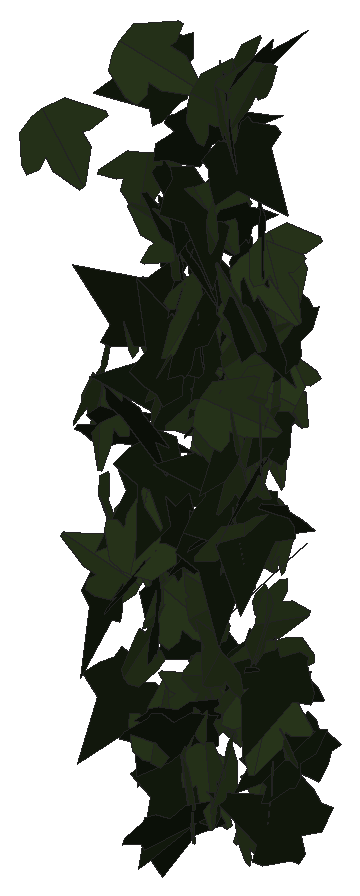
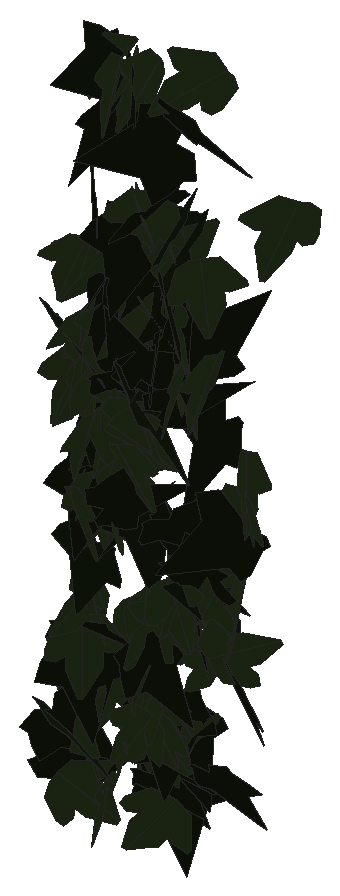
# SketchUp Ruby script. Lengths in inches.
U = 1.inch
M = Sketchup.active_model
def pt(a) = Geom::Point3d.new(a.map { |v| v * U })
def face(e, loops, mat)
  f = e.add_face(loops[0].map { |a| pt(a) })
  loops[1..].each { |l| e.add_face(l.map { |a| pt(a) }).erase! }
  f.material = f.back_material = mat if mat
  f
end
# faces: each face lists its corners as indices into pts; further lists are holes
def faces(e, pts, list, mat = nil) = list.each { |f| face(e, (f[0].is_a?(Array) ? f : [f]).map { |l| l.map { |i| pts[i] } }, mat) }
# xy, xz, yz: faces in a plane at the given z, y or x. An outline is a flat list of corners, or four numbers for a rectangle; further outlines are holes
def ring(l) = l.size == 4 ? [[l[0], l[1]], [l[2], l[1]], [l[2], l[3]], [l[0], l[3]]] : l.each_slice(2).to_a
def flat(e, list, mat, &to3) = list.each { |f| face(e, (f[0].is_a?(Array) ? f : [f]).map { |l| ring(l).map { |u, v| to3.(u, v) } }, mat) }
def xy(e, z, list, mat = nil) = flat(e, list, mat) { |x, y| [x, y, z] }
def xz(e, y, list, mat = nil) = flat(e, list, mat) { |x, z| [x, y, z] }
def yz(e, x, list, mat = nil) = flat(e, list, mat) { |y, z| [x, y, z] }
def lines(e, pts, list) = list.each { |a, b| e.add_line(pt(pts[a]), pt(pts[b])) }
# prism: a flat outline (further loops are holes) pulled along v
def prism(e, loops, v, mat = nil)
  f = face(e, loops, mat); d = Geom::Vector3d.new(v.map { |x| x * U })
  f.pushpull(f.normal.samedirection?(d) ? d.length : -d.length)
end
def box(e, o, s, mat = nil) = prism(e, [[o, [o[0] + s[0], o[1], o[2]], [o[0] + s[0], o[1] + s[1], o[2]], [o[0], o[1] + s[1], o[2]]]], [0, 0, s[2]], mat)
def at(x, y, z, deg = 0) = Geom::Transformation.translation(pt([x, y, z])) * Geom::Transformation.rotation(ORIGIN, Z_AXIS, deg.degrees)
def axes(o, x, y, z) = Geom::Transformation.new([*x, 0, *y, 0, *z, 0, *pt(o).to_a, 1])
def part(name) = M.definitions.add(name)
# library, detail: a bought-in or finely detailed component or shape, given as its bounding box
def library(name, o, s) = part(name).tap { |d| box(d.entities, o, s) }
def detail(e, o, s) = box(e.add_group.entities, o, s)
def put(e, d, t, mat = nil) = e.add_instance(d, t).tap { |i| i.material = mat if mat }
def group(e, t, mat = nil) = e.add_group.tap { |g| g.transformation = t; g.material = mat if mat }.entities
root = M.entities
M.materials.add("efeu1").color = [18, 25, 13]
M.materials.add("efeu2").color = [43, 57, 29]
c1 = part("ivyleaf_9")
p = [[1.54,2.16,1.25],[1.36,2.04,1.19],[-0.21,0.99,0.68],[-0.71,1.11,0.82],[-0.85,0.86,0.67],[-0.8,0.17,0.21],
  [-0.9,-0.01,0.1],[-0.67,-0.16,-0.02],[-0.08,-0.08,-0.05],[-0.03,-0.6,-0.4],[0.65,-0.88,-0.66],[0.83,-0.6,-0.49],
  [1.29,-0.42,-0.43],[1.8125,-0.07,-0.26],[1.21,0.44,0.15]]
faces(c1.entities,p,[[0,1,2,3,4,5,6,7,8,9,10,11,12,13,14]],"efeu1")
c2 = part("ivyleaf_10")
p = [[0,0.5,-0.03],[-0.0625,2.02,-0.43],[-0.19,2.01,-0.46],[-0.54,1.05,-0.29],[-0.52,0.625,-0.18],[-0.83,0.76,-0.28],
  [-1.16,0.64,-0.33],[-1.15,0.33,-0.24],[-0.77,-0.39,0.02],[-0.3,-0.51,0.16],[0.04,-0.48,0.23],[-0.02,2.01,-0.4375],
  [-0.06,2.01,-0.43],[0.04,-0.49,0.23],[0.67,-0.49,0.14],[1.38,0.36,-0.2],[1.375,0.51,-0.24],[0.81,0.65,-0.19],
  [0.62,0.59,-0.15],[0.6,1.09,-0.28],[0.5,1.23,-0.31]]
faces(c2.entities,p,[[0,1,2,3,4,5,6,7,8,9,10],[11,12,0,13,14,15,16,17,18,19,20]],"efeu2")
put(root,c1,axes([597.17,133.51,184.68],[0.19344,0.78927,-0.31319],[-0.07682,-0.30363,-0.81262],[-0.84566,0.20812,0.00218]))
put(root,c1,axes([597.22,133.8,197.03],[-0.33074,-0.73089,0.28254],[0.11402,0.25853,0.80224],[-0.77526,0.34984,-0.00255]))
put(root,c2,axes([598.65,133.66,205.125],[-0.33147,0.76317,-0.05677],[0.02262,-0.05207,-0.83204],[-0.76494,-0.33224,-0.00001]))
put(root,c1,axes([598.06,134.29,192.28],[0.09224,-0.89011,0.23083],[0.02783,-0.22918,-0.89487],[0.91914,0.09626,0.00393]))
put(root,c2,axes([596.73,133.97,196.96],[0.36238,-0.84765,0.07309],[0.03386,-0.06501,-0.92184],[0.85012,0.36391,0.00557]))
put(root,c1,axes([595.71,133.54,195.63],[0.79787,0.04653,-0.34518],[-0.34406,-0.02892,-0.79918],[-0.05418,0.86885,-0.00812]))
put(root,c2,axes([596.19,133.4,205.63],[0.32603,0.37985,0.79426],[0.47436,0.63773,-0.49971],[-0.7417,0.57484,0.02954]))
put(root,c1,axes([598.14,134.25,204.97],[0.01634,-0.07031,-0.84134],[0.83164,-0.14369,0.02816],[-0.14551,-0.82914,0.06646]))
put(root,c1,axes([598.95,134.2,193.69],[-0.38224,-0.75949,-0.28995],[0.16171,0.24297,-0.8496],[0.79671,-0.41369,0.03334]))
put(root,c2,axes([599.41,133.78,198.8],[-0.68374,0.33028,-0.53436],[-0.48633,0.22162,0.75927],[0.39762,0.839,0.0098]))
put(root,c2,axes([597.57,134.4,201.07],[0.01121,-0.17778,-0.85341],[0.47011,-0.7175,0.15564],[-0.7341,-0.4622,0.08664]))
put(root,c2,axes([593.4375,133.54,202.57],[0.43362,0.73756,0.41788],[0.06795,0.43763,-0.84292],[-0.84499,0.41369,0.14666]))
put(root,c1,axes([596.05,134.34,197.8],[0.16484,0.03859,0.90855],[-0.8719,-0.2556,0.16904],[0.25833,-0.8873,-0.00918]))
put(root,c2,axes([596.96,134.32,200.34],[-0.49306,-0.19256,-0.65801],[-0.57053,-0.33422,0.52531],[-0.3802,0.75125,0.06504]))
put(root,c2,axes([595.79,133.85,191.36],[0.8262,0.16039,-0.09412],[0.09089,0.02566,0.84159],[0.16224,-0.83115,0.00782]))
put(root,c2,axes([598.23,133.4,205.06],[0.01695,0.52,0.68475],[-0.19293,0.66972,-0.50381],[-0.83789,-0.14369,0.12985]))
put(root,c2,axes([599.07,133.98,193.07],[-0.43575,-0.80714,-0.07981],[0.04881,0.06434,-0.91717],[0.8096,-0.43831,0.01234]))
put(root,c2,axes([599.13,134.33,205.61],[-0.08859,-0.71936,0.36185],[-0.03531,-0.36021,-0.72475],[0.80446,-0.09503,0.00804]))
put(root,c2,axes([596.08,133.56,188.625],[0.1876,-0.54419,0.68042],[-0.2028,0.64962,0.57548],[-0.84734,-0.27596,0.01291]))
put(root,c1,axes([599.04,133.74,203.9],[0.12591,-0.45757,-0.69364],[-0.21384,0.66008,-0.47425],[0.80298,0.24754,-0.01753]))
put(root,c1,axes([596.8,134.53,196.1],[-0.32515,-0.07178,0.756],[-0.67039,-0.3592,-0.32243],[0.35674,-0.74043,0.08313]))
put(root,c2,axes([598.5625,133.56,196.59],[0.31512,0.26551,0.76924],[0.35454,0.69771,-0.38606],[-0.73249,0.45193,0.14408]))
put(root,c1,axes([596.55,134.64,201.24],[0.09239,-0.56269,0.59128],[0.12989,-0.57733,-0.56972],[0.80583,0.15758,0.02404]))
put(root,c1,axes([599.37,134.23,194.88],[-0.46831,0.47847,-0.45991],[0.30892,-0.34103,-0.66935],[-0.58738,-0.56083,0.01465]))
put(root,c1,axes([597.77,133.64,197.98],[-0.25926,0.53962,0.66936],[-0.4009,0.5426,-0.59271],[-0.76059,-0.46993,0.08425]))
put(root,c1,axes([596.28,134.29,200.88],[0.65973,-0.63387,0.08771],[0.06311,-0.06091,-0.9149],[0.63679,0.66274,-0.00019]))
put(root,c2,axes([598.71,134.17,195.99],[-0.30812,0.74007,-0.17715],[0.07386,-0.16113,-0.80163],[-0.75738,-0.31679,-0.00611]))
put(root,c1,axes([596.51,133.78,190.06],[-0.16401,0.14057,-0.81785],[-0.80945,0.15657,0.18924],[0.18283,0.81931,0.10416]))
put(root,c2,axes([597.125,134.18,185.7],[-0.52445,0.67905,-0.13617],[-0.00111,-0.17162,-0.85161],[-0.69257,-0.51394,0.10447]))
put(root,c2,axes([597.5,134.34,186.07],[0.67909,-0.21797,0.37866],[0.38147,-0.0454,-0.71026],[0.21301,0.77619,0.06479]))
put(root,c1,axes([596.69,134.18,186.85],[0.11997,0.66516,-0.5349],[-0.16394,-0.51214,-0.67363],[-0.83766,0.19549,0.05523]))
put(root,c2,axes([598.03,134.75,186.15],[-0.08182,0.24007,-0.78209],[0.1356,-0.77114,-0.2509],[-0.80679,-0.15396,0.03714]))
put(root,c2,axes([598.3125,134.55,192.98],[0.31203,-0.41931,0.67242],[0.65243,-0.27426,-0.47377],[0.44979,0.68869,0.22074]))
put(root,c2,axes([598.28,134.04,189.34],[-0.6344,0.11559,0.54828],[-0.53924,0.09913,-0.64485],[-0.15228,-0.83262,-0.00066]))
put(root,c1,axes([596.93,134.62,185.24],[-0.76967,-0.37313,-0.11884],[0.1206,0.02348,-0.85478],[0.37257,-0.77843,0.03118]))
put(root,c2,axes([599.02,133.86,194.97],[-0.0018,-0.64385,-0.59161],[0.02941,0.59123,-0.64353],[0.87389,-0.02122,0.02044]))
put(root,c1,axes([595.53,133.67,190.4],[-0.24967,0.76452,-0.27388],[-0.08823,0.2593,0.80425],[0.80729,0.26478,0.00319]))
put(root,c1,axes([597.36,134.59,201.79],[0.02343,-0.83752,-0.09939],[-0.00566,0.09927,-0.83785],[0.84338,0.02394,-0.00286]))
put(root,c1,axes([598.03,133.96,192.67],[-0.15279,0.91899,-0.03563],[0.00123,-0.03592,-0.93159],[-0.91968,-0.15273,0.00467]))
put(root,c2,axes([597.34,134.62,198.8],[0.35778,0.60825,-0.53666],[-0.33189,-0.42542,-0.70344],[-0.74014,0.48479,0.05602]))
put(root,c1,axes([596.59,134.4,204.74],[-0.73716,0.29395,0.34517],[-0.33352,0.0947,-0.79294],[-0.3071,-0.80844,0.03261]))
put(root,c2,axes([597.92,134.39,195.93],[-0.53778,-0.74544,-0.00437],[0.00148,0.00432,-0.91918],[0.74545,-0.53778,-0.00132]))
put(root,c1,axes([598.88,134.2,199.23],[0.53349,-0.5158,-0.46393],[-0.29057,0.3653,-0.74028],[0.62996,0.60531,0.05143]))
put(root,c1,axes([599.04,134.8,196.04],[-0.79129,-0.35342,0.00301],[-0.00249,-0.00181,-0.86663],[0.35342,-0.79129,0.00064]))
put(root,c2,axes([596.17,134,186.18],[0.10755,0.60025,-0.47323],[0.01256,0.47644,0.60717],[0.76425,-0.0923,0.05662]))
put(root,c1,axes([596.97,134.14,191.76],[-0.06208,0.04842,0.85915],[-0.50801,0.6932,-0.07578],[-0.69456,-0.51134,-0.02136]))
put(root,c2,axes([598.04,134.95,192.93],[0.30602,-0.59104,0.59331],[0.37138,-0.47039,-0.66015],[0.75061,0.4737,0.08474]))
put(root,c2,axes([597.49,134.34,201.66],[-0.74202,-0.33576,-0.3258],[0.30594,0.11391,-0.81419],[0.35395,-0.80235,0.02074]))
put(root,c2,axes([596.09,135.15,189.98],[-0.03052,-0.0414,0.8464],[0.3154,-0.78666,-0.0271],[0.78653,0.31384,0.04371]))
put(root,c2,axes([599.03,134.78,195.8],[-0.23433,0.61191,-0.44511],[0.11339,-0.43231,-0.654],[-0.74813,-0.25718,0.0403]))
put(root,c1,axes([598.78,134.95,200.67],[-0.04485,0.17328,0.80831],[0.10814,-0.80131,0.17778],[0.81957,0.11521,0.02077]))
put(root,c2,axes([598.4375,134.47,194.54],[-0.83738,0.33801,-0.11026],[0.09947,-0.04813,-0.90299],[-0.34134,-0.84323,0.00734]))
put(root,c1,axes([597.1,133.91,203.55],[0.08793,0.50047,-0.73814],[0.09525,0.7322,0.50779],[0.8867,-0.12828,0.01865]))
put(root,c2,axes([596.76,134.24,200.04],[0.03605,0.11079,0.8386],[-0.77799,0.33385,-0.01066],[-0.33207,-0.77013,0.11602]))
put(root,c1,axes([597.77,134.67,196.76],[-0.08956,0.66133,0.61469],[0.04767,-0.61338,0.66686],[0.90162,0.09812,0.0258]))
put(root,c1,axes([596.84,134.21,187.29],[0.36646,0.77889,-0.21045],[-0.22543,-0.12309,-0.84811],[-0.77469,0.40427,0.14724]))
put(root,c2,axes([598.11,134.72,195.17],[0.87973,0.10692,0.00564],[0.00533,0.00285,-0.88621],[-0.10694,0.87975,0.00218]))
put(root,c2,axes([599.03,134.5625,193.02],[-0.43766,-0.62456,-0.21132],[0.12303,0.17183,-0.76263],[0.64776,-0.45462,0.00207]))
put(root,c1,axes([597.92,134.82,198.45],[0.53965,-0.04797,0.72193],[-0.68136,0.26928,0.52721],[-0.2434,-0.86017,0.12479]))
put(root,c1,axes([596.04,135.21,193.43],[-0.47967,-0.73241,0.04364],[-0.03329,-0.03036,-0.87543],[0.73295,-0.48069,-0.0112]))
put(root,c2,axes([599.1,134.8,187.93],[0.74922,0.41322,-0.10648],[-0.10444,-0.03105,-0.85531],[-0.41375,0.75612,0.02307]))
put(root,c1,axes([596.33,134.44,200.16],[0.38454,0.0148,-0.82165],[-0.82147,0.03215,-0.38388],[0.02285,0.90661,0.02703]))
put(root,c2,axes([597.4,134.71,190.09],[-0.47977,-0.03468,0.59494],[-0.59169,-0.0634,-0.48085],[0.0711,-0.76165,0.01294]))
put(root,c2,axes([599.07,134.74,190.49],[0.53351,-0.67388,-0.24012],[-0.13939,0.19588,-0.85943],[0.70168,0.55129,0.01185]))
put(root,c1,axes([597.52,134.66,196.28],[-0.62472,0.63506,0.01941],[-0.01437,0.01309,-0.89083],[-0.6352,-0.62488,0.00106]))
put(root,c1,axes([599.05,134.48,193.41],[0.58217,0.48394,-0.23634],[-0.17986,-0.15335,-0.75704],[-0.50764,0.60932,-0.00282]))
put(root,c2,axes([598.7,134.25,197.61],[0.07169,-0.3433,0.75552],[0.06549,0.75831,0.33836],[-0.82727,0.03028,0.09226]))
put(root,c2,axes([597,135.26,187.84],[-0.22033,0.35121,0.67401],[0.27943,-0.61518,0.41189],[0.7068,0.35269,0.04727]))
put(root,c1,axes([599.15,135.17,189.04],[-0.68374,-0.45971,-0.23375],[0.19405,0.13031,-0.82391],[0.47782,-0.71074,0.00013]))
put(root,c1,axes([596.84,134.37,199.4],[-0.32059,0.10626,-0.83579],[-0.79461,0.25911,0.33774],[0.28005,0.85684,0.00152]))
put(root,c2,axes([598.77,134.41,196.7],[-0.24245,-0.355,-0.68162],[0.40616,0.54758,-0.42966],[0.65243,-0.47281,0.01418]))
put(root,c2,axes([595.36,134.5,197.81],[-0.16513,0.84579,0.30778],[-0.0943,0.29494,-0.86109],[-0.8951,-0.18711,0.03393]))
put(root,c2,axes([593.99,134.63,195.39],[0.15426,-0.7562,-0.4352],[-0.09219,0.42535,-0.77176],[0.8676,0.17965,-0.00463]))
put(root,c2,axes([599.25,135.11,196.41],[0.17714,0.36079,0.69796],[-0.52522,-0.47775,0.38026],[0.58435,-0.53877,0.1302]))
put(root,c1,axes([598.8,134.18,205.35],[0.27941,0.27983,0.73362],[0.29,0.68685,-0.37244],[-0.72966,0.38014,0.1329]))
put(root,c1,axes([599.75,135.16,184.5],[-0.13826,0.03219,0.81843],[-0.81374,-0.09986,-0.13354],[0.09322,-0.824,0.04815]))
put(root,c2,axes([594.48,135.09,189.85],[0.362,0.25231,0.76167],[-0.65545,-0.38899,0.44037],[0.46281,-0.74825,0.0279]))
put(root,c1,axes([597.77,134.49,201.06],[0.40961,0.72474,-0.05077],[-0.0265,-0.04333,-0.83248],[-0.72604,0.41046,0.00175]))
put(root,c2,axes([598.52,134.49,205.4375],[-0.18584,0.60569,0.53252],[-0.36004,0.42669,-0.61097],[-0.72167,-0.36884,0.16768]))
put(root,c2,axes([593.86,135.07,194.53],[-0.81376,0.32533,-0.09594],[-0.0403,-0.34034,-0.81227],[-0.33678,-0.74537,0.32902]))
put(root,c2,axes([596.58,135.02,187.13],[0.78688,-0.39093,-0.10725],[-0.08161,0.07663,-0.87805],[0.39708,0.79045,0.03208]))
put(root,c2,axes([596.25,134.58,197.43],[-0.42592,0.65941,0.36634],[-0.18045,0.31942,-0.78476],[-0.73244,-0.46215,-0.01968]))
put(root,c1,axes([597.7,135.49,197.34],[-0.45959,-0.64323,0.16682],[-0.09957,-0.13388,-0.79054],[0.657,-0.47025,-0.00312]))
put(root,c2,axes([596.47,134.64,198.89],[0.29155,-0.21377,-0.73495],[-0.46085,0.5789,-0.3512],[0.61112,0.53854,0.08578]))
put(root,c1,axes([593.91,135.24,189.38],[-0.67458,0.10769,-0.48965],[0.48782,-0.04845,-0.68271],[-0.11571,-0.83215,-0.02362]))
put(root,c2,axes([594.65,135.21,191.54],[0.65778,-0.11396,0.55782],[0.54534,-0.11876,-0.66733],[0.16357,0.85425,-0.01835]))
put(root,c2,axes([596.85,135.23,187.1875],[-0.54028,-0.30081,0.60182],[-0.49183,-0.3501,-0.61653],[0.45911,-0.72906,0.04775]))
put(root,c2,axes([598.625,134.93,187.78],[-0.8324,-0.2349,-0.07855],[0.07334,0.02929,-0.86487],[0.23658,-0.83558,-0.00823]))
put(root,c2,axes([598.71,135.27,185.625],[0.55474,-0.4199,0.3753],[0.33505,-0.17736,-0.69367],[0.45267,0.64585,0.0535]))
put(root,c2,axes([596.48,134.58,190.04],[0.31359,0.53986,0.63798],[0.2574,0.5859,-0.62231],[-0.79512,0.40259,0.05016]))
put(root,c2,axes([594.1875,134.73,191.8],[-0.57858,0.56927,0.3834],[-0.27418,0.26799,-0.81168],[-0.62919,-0.64026,0.00114]))
put(root,c2,axes([596.27,135.03,191.07],[-0.64219,-0.09933,0.44384],[-0.44118,-0.05057,-0.64967],[0.11052,-0.779,-0.01442]))
put(root,c2,axes([597.625,135.19,195.46],[0.43282,0.00626,-0.70011],[-0.70004,-0.00997,-0.43287],[-0.01177,0.82303,0.00008]))
put(root,c1,axes([597.1,134.79,197.16],[0.09893,-0.36904,0.7982],[-0.08205,0.79585,0.37813],[-0.87554,-0.11628,0.05475]))
put(root,c2,axes([598.77,134.91,199.96],[0.53831,0.36013,0.5195],[0.41949,0.30691,-0.64744],[-0.47286,0.68225,0.01703]))
put(root,c2,axes([597.98,135.28,195.64],[-0.38626,-0.16286,0.72061],[-0.64782,-0.31623,-0.41871],[0.35514,-0.75397,0.01996]))
put(root,c2,axes([596.8,135.22,187.93],[-0.55246,0.36477,-0.55973],[0.47883,-0.29033,-0.66182],[-0.46592,-0.73091,-0.01646]))
put(root,c2,axes([598.41,134.78,184.47],[-0.26203,0.54228,0.46518],[-0.22186,0.40923,-0.60202],[-0.67915,-0.34291,0.01719]))
put(root,c1,axes([595.41,135.54,192.37],[-0.77219,-0.18682,0.08903],[-0.08576,-0.02414,-0.79446],[0.18835,-0.77693,0.00328]))
put(root,c1,axes([594.45,135.51,186.58],[-0.78836,-0.19067,-0.09418],[0.0917,0.02148,-0.81109],[0.19187,-0.79368,0.00067]))
put(root,c1,axes([599.0625,134.63,191.36],[0.09449,0.71858,0.40246],[-0.07677,0.41102,-0.71584],[-0.82002,0.04433,0.11339]))
put(root,c2,axes([599.28,135.17,192.83],[0.54872,-0.41215,-0.40656],[-0.32659,0.24214,-0.68626],[0.47801,0.63856,-0.00218]))
put(root,c1,axes([596.89,135.25,189.1875],[0.14489,0.20474,-0.75608],[-0.61544,-0.4459,-0.23868],[-0.48456,0.62755,0.07708]))
put(root,c2,axes([598.14,134.88,198.54],[0.11885,0.75242,0.4757],[0.02291,0.47718,-0.76048],[-0.88989,0.11277,0.04395]))
put(root,c1,axes([597.8,135.82,199.44],[-0.0617,0.06059,-0.81283],[0.59774,-0.55082,-0.08643],[-0.55414,-0.60091,-0.00273]))
put(root,c1,axes([597.73,135.77,193.45],[-0.28527,-0.11319,0.73747],[-0.68625,-0.27006,-0.30691],[0.29282,-0.74318,-0.0008]))
put(root,c1,axes([598.93,135.18,188.47],[0.36906,0.58354,-0.42423],[-0.21833,-0.36384,-0.6904],[-0.68762,0.42872,-0.00848]))
put(root,c2,axes([598.89,135.36,189.15],[-0.58436,-0.63034,0.00049],[0.00572,-0.00597,-0.8595],[0.63032,-0.58433,0.00825]))
put(root,c2,axes([598.875,135.3,196.96],[-0.76489,-0.27888,-0.30823],[0.30082,0.0741,-0.81355],[0.28686,-0.82133,0.03127]))
put(root,c1,axes([597.02,135.3,197.36],[-0.51874,0.05791,0.59778],[0.57303,-0.18876,0.51555],[0.1798,0.76864,0.08157]))
put(root,c2,axes([598.89,135.85,184.9],[-0.37186,-0.40672,0.63951],[-0.31115,-0.56761,-0.54192],[0.69107,-0.47442,0.10011]))
put(root,c2,axes([594.84,135.5,201.18],[-0.54982,-0.60104,0.10204],[-0.0631,-0.08057,-0.81455],[0.60637,-0.55337,0.00776]))
put(root,c1,axes([599.41,135.79,186.8125],[0.01237,0.1874,-0.74979],[-0.12313,-0.73983,-0.18694],[-0.76298,0.12243,0.01801]))
put(root,c2,axes([599.01,135.24,200.4375],[0.31513,0.67535,0.25993],[0.10186,0.23929,-0.7452],[-0.71644,0.33107,0.00839]))
put(root,c1,axes([593.83,134.99,193.82],[0.75564,0.25005,0.36282],[0.32071,0.18181,-0.79325],[-0.30217,0.81827,0.06538]))
put(root,c2,axes([598.74,135.28,195.31],[-0.15209,0.78695,0.1091],[-0.03618,0.1041,-0.80136],[-0.79365,-0.15555,0.01563]))
put(root,c2,axes([599.18,135.36,186.37],[-0.60879,0.32931,-0.52967],[-0.48882,0.20777,0.69102],[0.38736,0.77975,0.03957]))
put(root,c2,axes([596.09,135.47,184.92],[-0.66372,-0.23206,-0.5165],[0.55122,-0.08268,-0.67118],[0.12958,-0.83694,0.20952]))
put(root,c1,axes([599.6875,135.28,198.05],[-0.49909,0.51412,0.30207],[-0.22136,0.20602,-0.71639],[-0.55368,-0.54579,0.01413]))
put(root,c2,axes([598.91,134.91,190.21],[-0.10059,-0.31156,-0.81234],[0.19601,0.78861,-0.32673],[0.84767,-0.21932,-0.02084]))
put(root,c2,axes([599.24,134.98,196.29],[-0.0136,-0.2923,-0.72557],[0.02358,0.7252,-0.29259],[0.78188,-0.02696,-0.0038]))
put(root,c2,axes([597.25,135.55,195.01],[0.69061,-0.20392,-0.30723],[-0.29605,0.08228,-0.72007],[0.21984,0.75137,-0.00453]))
put(root,c2,axes([598.84,135.51,198.49],[0.08253,0.76939,-0.10646],[-0.02976,-0.10384,-0.77358],[-0.77615,0.08579,0.01835]))
put(root,c1,axes([599.65,135.31,186.34],[-0.48512,0.61271,0.34592],[-0.34613,0.158,-0.76528],[-0.61259,-0.57449,0.15846]))
put(root,c2,axes([596.75,135.51,187.22],[-0.65289,0.02002,-0.38554],[0.3828,-0.06458,-0.65161],[-0.05003,-0.75547,0.04548]))
